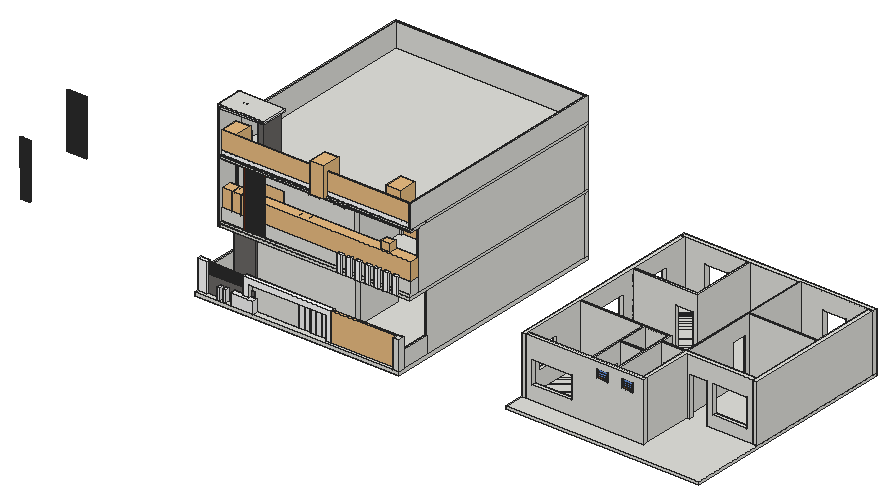
# SketchUp Ruby script. Lengths in inches.
U = 1.inch
M = Sketchup.active_model
def pt(a) = Geom::Point3d.new(a.map { |v| v * U })
def face(e, loops, mat)
  f = e.add_face(loops[0].map { |a| pt(a) })
  loops[1..].each { |l| e.add_face(l.map { |a| pt(a) }).erase! }
  f.material = f.back_material = mat if mat
  f
end
# faces: each face lists its corners as indices into pts; further lists are holes
def faces(e, pts, list, mat = nil) = list.each { |f| face(e, (f[0].is_a?(Array) ? f : [f]).map { |l| l.map { |i| pts[i] } }, mat) }
# xy, xz, yz: faces in a plane at the given z, y or x. An outline is a flat list of corners, or four numbers for a rectangle; further outlines are holes
def ring(l) = l.size == 4 ? [[l[0], l[1]], [l[2], l[1]], [l[2], l[3]], [l[0], l[3]]] : l.each_slice(2).to_a
def flat(e, list, mat, &to3) = list.each { |f| face(e, (f[0].is_a?(Array) ? f : [f]).map { |l| ring(l).map { |u, v| to3.(u, v) } }, mat) }
def xy(e, z, list, mat = nil) = flat(e, list, mat) { |x, y| [x, y, z] }
def xz(e, y, list, mat = nil) = flat(e, list, mat) { |x, z| [x, y, z] }
def yz(e, x, list, mat = nil) = flat(e, list, mat) { |y, z| [x, y, z] }
def lines(e, pts, list) = list.each { |a, b| e.add_line(pt(pts[a]), pt(pts[b])) }
# prism: a flat outline (further loops are holes) pulled along v
def prism(e, loops, v, mat = nil)
  f = face(e, loops, mat); d = Geom::Vector3d.new(v.map { |x| x * U })
  f.pushpull(f.normal.samedirection?(d) ? d.length : -d.length)
end
def box(e, o, s, mat = nil) = prism(e, [[o, [o[0] + s[0], o[1], o[2]], [o[0] + s[0], o[1] + s[1], o[2]], [o[0], o[1] + s[1], o[2]]]], [0, 0, s[2]], mat)
def at(x, y, z, deg = 0) = Geom::Transformation.translation(pt([x, y, z])) * Geom::Transformation.rotation(ORIGIN, Z_AXIS, deg.degrees)
def axes(o, x, y, z) = Geom::Transformation.new([*x, 0, *y, 0, *z, 0, *pt(o).to_a, 1])
def part(name) = M.definitions.add(name)
# library, detail: a bought-in or finely detailed component or shape, given as its bounding box
def library(name, o, s) = part(name).tap { |d| box(d.entities, o, s) }
def detail(e, o, s) = box(e.add_group.entities, o, s)
def put(e, d, t, mat = nil) = e.add_instance(d, t).tap { |i| i.material = mat if mat }
def group(e, t, mat = nil) = e.add_group.tap { |g| g.transformation = t; g.material = mat if mat }.entities
root = M.entities
M.materials.add("Paint Brown Gloss 1.5cm").color = [255, 255, 255]
M.materials.add("Polis06_194").color = [79, 50, 36]
M.materials.add("Stone C 250cm").color = [107, 104, 102]
M.materials.add("Tiles Marble White 03 180cm\#1").color = [241, 241, 241]
M.materials.add("Wood Dark 02 100cm").color = [99, 39, 19]
M.materials.add("Wood Mahogany 33-46 100cm").color = [84, 42, 21]
M.materials.add("[Translucent Glass Blue]").color = [100, 149, 237]
M.materials["[Translucent Glass Blue]"].alpha = 0.5
M.materials.add("[Translucent Glass Gray]").color = [128, 128, 128]
M.materials["[Translucent Glass Gray]"].alpha = 0.1
M.materials.add("[Wood Floor Parquet]").color = [145, 89, 39]
c1 = part("Stair step")
box(c1.entities,[0,0,0],[42,12,7])
c2 = part("ventilater")
prism(c2.entities,[[[2,7.78,8.95],[2,1.41,2.59],[2,0,4],[2,6.36,10.36]]],[20,0,0],"[Translucent Glass Blue]")
prism(c2.entities,[[[2,1.41,13.34],[22,1.41,13.34],[22,0,14.75],[2,0,14.75]]],[0,6.36,6.36],"[Translucent Glass Blue]")
prism(c2.entities,[[[2,1.41,7.96],[22,1.41,7.96],[22,0,9.375],[2,0,9.375]]],[0,6.36,6.36],"[Translucent Glass Blue]")
g1 = group(c2.entities,at(0,0,0))
xy(g1,0,[[0,0,24,9]],"[Wood Floor Parquet]")
xy(g1,2,[[2,0,22,9]],"[Wood Floor Parquet]")
xy(g1,22,[[2,0,22,9]],"[Wood Floor Parquet]")
xy(g1,24,[[0,0,24,9]],"[Wood Floor Parquet]")
xz(g1,0,[[[0,0,24,24],[2,2,22,22]]],"[Wood Floor Parquet]")
xz(g1,9,[[[0,0,24,24],[2,2,22,22]]],"[Wood Floor Parquet]")
yz(g1,0,[[0,0,9,24]],"[Wood Floor Parquet]")
yz(g1,2,[[0,2,9,22]],"[Wood Floor Parquet]")
yz(g1,22,[[0,2,9,22]])
yz(g1,24,[[0,0,9,24]],"[Wood Floor Parquet]")
c3 = library("PINTU 6 YA",[0,-0.6875,0],[35.83,8.07,80.71])
c4 = library("Flush door assembly",[0,0,0],[5.12,30.08,83.9375])
c5 = part("Flush door")
xy(c5.entities,0,[[0,0,4.72,1.18],[0,34.25,4.72,35.43]],"Polis06_194")
xy(c5.entities,85.26,[[0,1.18,4.72,34.25]],"Polis06_194")
xy(c5.entities,86.61,[[0,0,4.72,35.43]],"Polis06_194")
xz(c5.entities,0,[[0,0,4.72,86.61]],"Polis06_194")
xz(c5.entities,1.18,[[0,0,2.36,85.26],[2.36,0,4.72,85.26]],"Polis06_194")
xz(c5.entities,34.25,[[0,0,4.72,85.26]],"Polis06_194")
xz(c5.entities,35.43,[[0,0,4.72,86.61]],"Polis06_194")
yz(c5.entities,0,[[0,0,1.18,86.61],[34.25,0,35.43,86.61],[1.18,85.26,34.25,86.61]],"Polis06_194")
yz(c5.entities,2.36,[[1.18,0,34.25,0,34.25,85.21,1.18,85.26]],"Polis06_194")
yz(c5.entities,4.72,[[0,0,1.18,86.61],[34.25,0,35.43,86.61],[1.18,85.26,34.25,86.61]],"Polis06_194")
c6 = library("Untitled",[0,0,0],[36,4.39,84])
c7 = library("Window 46-12",[-37.28,-2.15,0],[74.56,4.3,92.91])
c8 = library("Window 46-47",[-61.02,-2.17,0],[122.04,4.34,74.02])
c9 = library("Window 46-15",[-34.06,-3.13,0],[68.12,6.24,59.06])
c10 = part("Flat panel")
box(c10.entities,[0,0,-1],[25,83.4375,1])
c11 = library("Round downlight",[0,0,-2.25],[6,6,4])
c12 = part("Square post")
box(c12.entities,[0,0,0],[1.8125,1.75,76.8125])
c13 = library("Garage Gate 243 111",[-105.76,-3.7,0],[211.52,7.4,101.23])
c14 = library("Potted Plant 02",[-16.98,-19.78,0],[30.04,38.68,37.52])
c15 = library("Potted Plant 13",[-10,-7.28,0],[18.93,15.17,39.22])
c16 = part("Group\#18")
p = [[1.37,4.61,43.28],[1.44,55.5625,43.28],[1.44,55.5625,4.4375],[1.37,4.61,4.4375]]
faces(c16.entities,p,[[0,1,2,3]],"[Translucent Glass Gray]")
g2 = group(c16.entities,at(0,0,0))
xy(g2,0,[[0.0625,0,2.5,60]])
xy(g2,3.125,[[0,3.125,0.59,56.875],[1.84,3.125,2.4375,56.875]])
xy(g2,4.4375,[[0.66,4.4375,1.91,55.5625]])
xy(g2,43.5625,[[0.66,4.4375,1.91,55.5625]])
xy(g2,44.875,[[0,3.125,0.59,56.875],[1.84,3.125,2.4375,56.875]])
xy(g2,48,[[0.0625,0,2.5,60]])
xz(g2,0,[[0.0625,0,2.5,48]])
xz(g2,3.125,[[0,3.125,0.59,44.875],[1.84,3.125,2.4375,44.875]])
xz(g2,4.4375,[[0.66,4.4375,1.91,43.5625]])
xz(g2,55.5625,[[0.66,4.4375,1.91,43.5625]])
xz(g2,56.875,[[0,3.125,0.59,44.875],[1.84,3.125,2.4375,44.875]])
xz(g2,60,[[0.0625,0,2.5,48]])
p = [[0,3.125,3.125],[0.0625,0,0],[0.0625,0,48],[0,3.125,44.875],[0,56.875,3.125],[0.0625,60,0],
  [2.5,0,0],[2.4375,3.125,3.125],[2.4375,3.125,44.875],[2.5,0,48],[2.5,60,0],[2.4375,56.875,3.125],
  [0,56.875,44.875],[0.0625,60,48],[2.5,60,48],[2.4375,56.875,44.875],[0.66,4.4375,4.4375],[0.59,3.125,3.125],
  [0.59,3.125,44.875],[0.66,4.4375,43.5625],[0.66,55.5625,4.4375],[0.59,56.875,3.125],[1.84,3.125,3.125],[1.91,4.4375,4.4375],
  [1.91,4.4375,43.5625],[1.84,3.125,44.875],[1.84,56.875,3.125],[1.91,55.5625,4.4375],[0.66,55.5625,43.5625],[0.59,56.875,44.875],
  [1.84,56.875,44.875],[1.91,55.5625,43.5625]]
faces(g2,p,[[0,1,2,3],[4,5,1,0],[6,7,8,9],[10,11,7,6],[12,13,5,4],[14,15,11,10],[16,17,18,19],[20,21,17,16],
  [22,23,24,25],[26,27,23,22],[28,29,21,20],[30,31,27,26],[19,18,29,28],[25,24,31,30],[3,2,13,12],[9,8,15,14]])
c17 = part("Group\#28")
xy(c17.entities,0,[[0,0,402.5,9]])
xy(c17.entities,36,[[51,0,99,9],[298.5,0,346.5,9]])
xy(c17.entities,84,[[51,0,99,9],[298.5,0,346.5,9]])
xy(c17.entities,120,[[0,0,402.5,9]])
xz(c17.entities,0,[[0,0,9,120],[[9,0,141,120],[51,36,99,84]],[141,0,145.5,120],[145.5,0,247,120],[247,0,251.5,120],
  [[251.5,0,393.5,120],[298.5,36,346.5,84]],[393.5,0,402.5,120]])
xz(c17.entities,9,[[[0,0,402.5,120],[51,36,99,84],[298.5,36,346.5,84]]])
yz(c17.entities,0,[[0,0,9,120]])
yz(c17.entities,51,[[0,36,9,84]])
yz(c17.entities,99,[[0,36,9,84]])
yz(c17.entities,298.5,[[0,36,9,84]])
yz(c17.entities,346.5,[[0,36,9,84]])
yz(c17.entities,402.5,[[0,0,9,120]])
c18 = part("Group\#29")
xy(c18.entities,0,[[0,0,9,416]])
xy(c18.entities,36,[[0,33,9,81],[0,183.5,9,255.5],[0,308,9,368]])
xy(c18.entities,84,[[0,33,9,81],[0,183.5,9,255.5],[0,308,9,368]])
xy(c18.entities,120,[[0,0,9,416]])
xz(c18.entities,0,[[0,0,9,120]])
xz(c18.entities,33,[[0,36,9,84]])
xz(c18.entities,81,[[0,36,9,84]])
xz(c18.entities,183.5,[[0,36,9,84]])
xz(c18.entities,255.5,[[0,36,9,84]])
xz(c18.entities,308,[[0,36,9,84]])
xz(c18.entities,368,[[0,36,9,84]])
xz(c18.entities,416,[[0,0,9,120]])
yz(c18.entities,0,[[[0,0,416,120],[183.5,36,255.5,84],[308,36,368,84],[33,36,81,84]]])
yz(c18.entities,9,[[0,0,9,120],[[9,0,141,120],[33,36,81,84]],[141,0,145.5,120],[[145.5,0,279.5,120],[183.5,36,255.5,84]],[279.5,0,284,120],
  [[284,0,416,120],[308,36,368,84]]])
c19 = part("Group\#30")
xy(c19.entities,0,[[0,0,246,9]])
xy(c19.entities,30,[[12,0,96,9]])
xy(c19.entities,78,[[12,0,96,9]])
xy(c19.entities,90,[[148.5,0,172.5,9],[201,0,225,9]])
xy(c19.entities,108,[[148.5,0,172.5,9],[201,0,225,9]])
xy(c19.entities,120,[[0,0,246,9]])
xz(c19.entities,0,[[[0,0,246,120],[12,30,96,78],[148.5,90,172.5,108],[201,90,225,108]]])
xz(c19.entities,9,[[[0,0,132,120],[12,30,96,78]],[132,0,136.5,120],[[136.5,0,184.5,120],[148.5,90,172.5,108]],[184.5,0,189,120],[[189,0,237,120],[201,90,225,108]],
  [237,0,246,120]])
yz(c19.entities,0,[[0,0,9,120]])
yz(c19.entities,12,[[0,30,9,78]])
yz(c19.entities,96,[[0,30,9,78]])
yz(c19.entities,148.5,[[0,90,9,108]])
yz(c19.entities,172.5,[[0,90,9,108]])
yz(c19.entities,201,[[0,90,9,108]])
yz(c19.entities,225,[[0,90,9,108]])
yz(c19.entities,246,[[0,0,9,120]])
c20 = part("Group\#33")
xy(c20.entities,0,[[0,0,90,4.5],[126,0,126,4.5,132,4.5,132,136.5,136.5,136.5,136.5,0]])
xy(c20.entities,84,[[90,0,126,4.5]])
xy(c20.entities,120,[[0,0,136.5,0,136.5,136.5,132,136.5,132,4.5,0,4.5]])
xz(c20.entities,0,[[0,0,90,0,90,84,126,84,126,0,136.5,0,136.5,120,0,120]])
xz(c20.entities,4.5,[[0,0,0,120,132,120,132,0,126,0,126,84,90,84,90,0]])
xz(c20.entities,136.5,[[132,0,136.5,120]])
yz(c20.entities,0,[[0,0,4.5,120]])
yz(c20.entities,90,[[0,0,4.5,84]])
yz(c20.entities,126,[[0,0,4.5,84]])
yz(c20.entities,132,[[4.5,0,136.5,120]])
yz(c20.entities,136.5,[[0,0,136.5,120]])
c21 = part("Group\#34")
xy(c21.entities,0,[[0,-157,4.55,-42],[0,-6,0,10.5,4.5,10.5,4.5,4.5,146.5,4.5,146.5,0,4.55,0,4.55,-6],[0,46.5,4.5,136.5]])
xy(c21.entities,84,[[0,-42,4.55,-6],[0,10.5,4.5,46.5]])
xy(c21.entities,120,[[0,-157,4.55,-157,4.55,0,146.5,0,146.5,4.5,4.5,4.5,4.5,136.5,0,136.5]])
xz(c21.entities,-157,[[0,0,4.55,120]])
xz(c21.entities,-42,[[0,0,4.55,84]])
xz(c21.entities,-6,[[0,0,4.55,84]])
xz(c21.entities,0,[[4.55,0,146.5,120]])
xz(c21.entities,4.5,[[4.5,0,146.5,120]])
xz(c21.entities,10.5,[[0,0,4.5,84]])
xz(c21.entities,46.5,[[0,0,4.5,84]])
xz(c21.entities,136.5,[[0,0,4.5,120]])
yz(c21.entities,0,[[-157,0,-157,120,136.5,120,136.5,0,46.5,0,46.5,84,10.5,84,10.5,0,-6,0,-6,84,-42,84,-42,0]])
yz(c21.entities,4.5,[[4.5,0,10.5,0,10.5,84,46.5,84,46.5,0,136.5,0,136.5,120,4.5,120]])
yz(c21.entities,4.55,[[-157,0,-42,0,-42,84,-6,84,-6,0,0,0,0,120,-157,120]])
yz(c21.entities,146.5,[[0,0,4.5,120]])
c22 = part("Group\#38")
xy(c22.entities,0,[[184.5,0,184.5,66,136.5,66,136.5,60,132,60,132,132,126,132,126,136.5,154.5,136.5,154.5,132,136.5,132,136.5,70.5,184.5,70.5,184.5,132,178.5,132,178.5,136.5,189,136.5,189,0],[132,0,136.5,30],[0,132,90,136.5]])
xy(c22.entities,84,[[132,30,136.5,60],[90,132,126,136.5],[154.5,132,178.5,136.5]])
xy(c22.entities,120,[[[132,0,136.5,0,136.5,66,184.5,66,184.5,0,189,0,189,136.5,0,136.5,0,132,132,132],[136.5,70.5,184.5,132]]])
xz(c22.entities,0,[[132,0,136.5,120],[184.5,0,189,120]])
xz(c22.entities,30,[[132,0,136.5,84]])
xz(c22.entities,60,[[132,0,136.5,84]])
xz(c22.entities,66,[[136.5,0,184.5,120]])
xz(c22.entities,70.5,[[136.5,0,184.5,120]])
xz(c22.entities,132,[[0,0,90,0,90,84,126,84,126,0,132,0,132,120,0,120],[136.5,0,154.5,0,154.5,84,178.5,84,178.5,0,184.5,0,184.5,120,136.5,120]])
xz(c22.entities,136.5,[[0,0,0,120,189,120,189,0,178.5,0,178.5,84,154.5,84,154.5,0,126,0,126,84,90,84,90,0]])
yz(c22.entities,0,[[132,0,136.5,120]])
yz(c22.entities,90,[[132,0,136.5,84]])
yz(c22.entities,126,[[132,0,136.5,84]])
yz(c22.entities,132,[[0,0,0,120,132,120,132,0,60,0,60,84,30,84,30,0]])
yz(c22.entities,136.5,[[0,0,30,0,30,84,60,84,60,0,66,0,66,120,0,120],[70.5,0,132,120]])
yz(c22.entities,154.5,[[132,0,136.5,84]])
yz(c22.entities,178.5,[[132,0,136.5,84]])
yz(c22.entities,184.5,[[0,0,66,120],[70.5,0,132,120]])
yz(c22.entities,189,[[0,0,136.5,120]])
c23 = part("Group\#39")
prism(c23.entities,[[[6,4.5,0],[0,4.5,0],[0,4.5,120],[48,4.5,120],[48,4.5,0],[30,4.5,0],[30,4.5,84],[6,4.5,84]]],[0,-4.5,0])
c24 = part("Group\#31")
xy(c24.entities,0,[[0,0,0,113.5,15,113.5,15,104.5,9,104.5,9,0],[51,104.5,147.5,113.5]])
xy(c24.entities,24,[[63.5,104.5,135.5,113.5]])
xy(c24.entities,84,[[15,104.5,51,113.5],[63.5,104.5,135.5,113.5]])
xy(c24.entities,120,[[0,0,9,0,9,104.5,147.5,104.5,147.5,113.5,0,113.5]])
xz(c24.entities,0,[[0,0,9,120]])
xz(c24.entities,104.5,[[[9,0,15,0,15,84,51,84,51,0,147.5,0,147.5,120,9,120],[63.5,24,135.5,84]]])
xz(c24.entities,113.5,[[[0,0,0,120,147.5,120,147.5,0,51,0,51,84,15,84,15,0],[63.5,24,135.5,84]]])
yz(c24.entities,0,[[0,0,113.5,120]])
yz(c24.entities,9,[[0,0,104.5,120]])
yz(c24.entities,15,[[104.5,0,113.5,84]])
yz(c24.entities,51,[[104.5,0,113.5,84]])
yz(c24.entities,63.5,[[104.5,24,113.5,84]])
yz(c24.entities,135.5,[[104.5,24,113.5,84]])
yz(c24.entities,147.5,[[104.5,0,113.5,120]])
c25 = part("Group\#19")
p = [[0.77,2.6,2.4375],[0.77,2.6,45.4375],[0.76,69.5625,45.4375],[0.76,69.5625,2.4375]]
faces(c25.entities,p,[[0,1,2,3]],"[Translucent Glass Gray]")
g3 = group(c25.entities,at(0,0,0))
xy(g3,0,[[0,0,1.5,72]])
xy(g3,1.6875,[[0,1.6875,0.32,70.3125],[1.13,1.6875,1.5,70.3125]])
xy(g3,2.4375,[[0.32,2.4375,1.13,69.5625]])
xy(g3,45.5625,[[0.32,2.4375,1.13,69.5625]])
xy(g3,46.3125,[[0,1.6875,0.32,70.3125],[1.13,1.6875,1.5,70.3125]])
xy(g3,48,[[0,0,1.5,72]])
xz(g3,0,[[0,0,1.5,48]])
xz(g3,1.6875,[[0,1.6875,0.32,46.3125],[1.13,1.6875,1.5,46.3125]])
xz(g3,2.4375,[[0.32,2.4375,1.13,45.5625]])
xz(g3,69.5625,[[0.32,2.4375,1.13,45.5625]])
xz(g3,70.3125,[[0,1.6875,0.32,46.3125],[1.13,1.6875,1.5,46.3125]])
xz(g3,72,[[0,0,1.5,48]])
yz(g3,0,[[[0,0,72,48],[1.6875,1.6875,70.3125,46.3125]]])
yz(g3,0.32,[[[1.6875,1.6875,70.3125,46.3125],[2.4375,2.4375,69.5625,45.5625]]])
yz(g3,1.13,[[[1.6875,1.6875,70.3125,46.3125],[2.4375,2.4375,69.5625,45.5625]]])
yz(g3,1.5,[[[0,0,72,48],[1.6875,1.6875,70.3125,46.3125]]])
c26 = part("Group\#40")
p = [[44.3125,1.21,43.61],[44.3125,1.21,3.6875],[3.84,1.24,3.6875],[3.84,1.24,43.61]]
faces(c26.entities,p,[[0,1,2,3]],"[Translucent Glass Gray]")
g4 = group(c26.entities,at(0,0,0))
xy(g4,0,[[0,0,48,2.6875]])
xy(g4,2.4375,[[2.4375,0,45.5625,0.78],[2.4375,1.85,45.5625,2.6875]])
xy(g4,3.6875,[[3.6875,0.78,44.3125,1.85]])
xy(g4,44.3125,[[3.6875,0.78,44.3125,1.85]])
xy(g4,45.5625,[[2.4375,0,45.5625,0.78],[2.4375,1.85,45.5625,2.6875]])
xy(g4,48,[[0,0,48,2.6875]])
xz(g4,0,[[[0,0,48,48],[2.4375,2.4375,45.5625,45.5625]]])
xz(g4,0.78,[[[2.4375,2.4375,45.5625,45.5625],[3.6875,3.6875,44.3125,44.3125]]])
xz(g4,1.85,[[[2.4375,2.4375,45.5625,45.5625],[3.6875,3.6875,44.3125,44.3125]]])
xz(g4,2.6875,[[[0,0,48,48],[2.4375,2.4375,45.5625,45.5625]]])
yz(g4,0,[[0,0,2.6875,48]])
yz(g4,2.4375,[[0,2.4375,0.78,45.5625],[1.85,2.4375,2.6875,45.5625]])
yz(g4,3.6875,[[0.78,3.6875,1.85,44.3125]])
yz(g4,44.3125,[[0.78,3.6875,1.85,44.3125]])
yz(g4,45.5625,[[0,2.4375,0.78,45.5625],[1.85,2.4375,2.6875,45.5625]])
yz(g4,48,[[0,0,2.6875,48]])
c27 = part("Round rod")
prism(c27.entities,[[[1.11,0.71,0],[1.125,0.5625,0],[1.11,0.42,0],[1.05,0.28,0],[0.96,0.16,0],[0.84,0.08,0],[0.71,0.02,0],[0.5625,0,0],[0.42,0.02,0],[0.28,0.08,0],[0.16,0.16,0],[0.08,0.28,0],[0.02,0.42,0],[0,0.5625,0],[0.02,0.71,0],[0.08,0.84,0],[0.16,0.96,0],[0.28,1.05,0],[0.42,1.11,0],[0.5625,1.125,0],[0.71,1.11,0],[0.84,1.05,0],[0.96,0.96,0],[1.05,0.84,0]]],[0,0,24])
c28 = library("Group\#45",[0,0,0],[399.29,21.95,36.98])
c29 = part("Vertical batten")
prism(c29.entities,[[[0,0.125,0],[1.6875,0.125,0],[1.6875,-0.5,0],[0,-0.5,0]]],[0,-0.125,115])
c30 = part("Group\#59")
xy(c30.entities,0,[[0,0.125,21.3,0.4375]])
xy(c30.entities,115,[[0,0,21.3,0.3125]])
yz(c30.entities,0,[[0.125,0,0,115,0.3125,115,0.4375,0]])
yz(c30.entities,21.3,[[0.125,0,0.4375,0,0.3125,115,0,115]])
p = [[21.3,0,115],[0.625,0,115],[0.625,0.125,0],[21.3,0.125,0],[0,0.3125,115],[21.3,0.3125,115],
  [21.3,0.4375,0],[0,0.4375,0]]
faces(c30.entities,p,[[0,1,2,3],[4,5,6,7]])
put(c30.entities,c29,at(0,0,0))
put(c30.entities,c29,at(3.92,0,0))
put(c30.entities,c29,at(7.85,0,0))
put(c30.entities,c29,at(11.77,0,0))
put(c30.entities,c29,at(15.69,0,0))
put(c30.entities,c29,at(19.61,0,0))
c31 = part("Group\#61")
prism(c31.entities,[[[9.625,2.75,0],[9.625,2.75,33.375],[9.625,7.8125,33.375],[9.625,8.875,33.375],[9.625,8.875,36.5625],[9.625,0,36.5625],[9.625,0,0]]],[-9.625,0,0])
c32 = library("Group\#62",[0,0,0],[397.4375,3.15,36.98])
box(root,[335.52,145.54,347.82],[95.87,55.93,0.79])
box(root,[413.77,151.7,252],[12,45.8,89.625],"Stone C 250cm")
prism(root,[[[311.52,611.04,0],[335.52,611.04,0],[335.52,606.54,0],[316.02,606.54,0],[316.02,132.1,0],[311.52,132.1,0]]],[0,0,36])
xy(root,-6.5625,[[947.33,195.04,1079.33,327.04],[1083.83,195.04,1131.83,261.04],[1083.83,265.54,1131.83,327.04],[947.33,470.04,1079.33,602.04],[1189.83,470.04,1331.83,602.04]])
xy(root,0,[[726.02,116.04,738.02,128.04],[733.52,128.04,738.02,188.04],[733.52,188.04,738.02,378.54],[344.52,197.04,476.52,329.04],[481.02,197.04,529.02,263.04],
  [481.02,267.54,476.52,329.04,529.02,329.04,529.02,267.54],[587.02,387.54,729.02,465.54],[344.52,470.04,476.52,602.04],[587.02,470.04,729.02,602.04]])
xy(root,36,[[733.52,128.04,738.02,188.04]])
xy(root,60,[[726.02,116.04,738.02,128.04]])
xy(root,126,[[344.52,195.04,476.52,327.04],[481.02,195.04,529.02,261.04],[481.02,265.54,529.02,327.04],[344.52,470.04,476.52,602.04],[587.02,470.04,729.02,602.04]])
xy(root,131,[[481.02,267.54,529.02,267.54,529.02,329.04,476.52,329.04]])
xy(root,252,[[340.02,145.54,738.02,146.54],[340.02,146.54,733.52,150.04],[733.52,146.54,738.02,611.04],[335.52,606.54,733.52,611.04]])
xy(root,255,[[340.02,145.54,738.02,146.54]])
xy(root,264,[[340.02,146.54,733.52,148.29],[340.02,148.29,733.52,150.04]])
xy(root,300.98,[[733.52,146.54,738.02,611.04],[335.52,606.54,733.52,611.04]])
xz(root,116.04,[[726.02,0,738.02,60]])
xz(root,128.04,[[726.02,0,733.52,60],[733.52,0,738.02,36],[733.52,36,738.02,60]])
xz(root,145.54,[[340.02,252,738.02,255]])
xz(root,146.54,[[340.02,252,733.52,255],[733.52,252,738.02,255],[733.52,255,738.02,300.98]])
xz(root,146.54,[[340.02,255,733.52,264]],"Paint Brown Gloss 1.5cm")
xz(root,150.04,[[340.02,252,733.52,264]])
xz(root,188.04,[[733.52,0,738.02,36]])
xz(root,267.54,[[481.02,0,529.02,131]])
xz(root,329.04,[[476.52,0,529.02,131]])
xz(root,606.54,[[335.52,252,733.52,300.98]])
xz(root,611.04,[[335.52,252,733.52,300.98],[733.52,252,738.02,300.98]])
yz(root,335.52,[[606.54,252,201.47,252.15,201.49,301.14,606.55,300.99,606.55,300.98,606.54,300.98],[606.54,252,606.54,300.98,606.55,300.98],[606.54,252,606.55,300.98,611.04,300.98,611.04,252]])
yz(root,340.02,[[145.54,252,146.54,255],[146.54,252,150.04,264],[606.54,252,606.55,300.99,201.49,301.14,201.47,252.15]])
yz(root,529.02,[[267.54,0,329.04,131]])
yz(root,726.02,[[116.04,0,128.04,60]])
yz(root,733.52,[[128.04,0,188.04,36],[146.54,252,150.04,264],[150.04,252,606.54,300.98],[606.54,252,611.04,300.98],[146.54,264,150.04,300.98]])
yz(root,738.02,[[116.04,0,128.04,60],[128.04,0,188.04,36],[145.54,252,146.54,255],[146.54,252,611.04,300.98]])
p = [[476.52,329.04,0],[481.02,267.54,0],[481.02,267.54,126],[481.02,267.54,131],[476.52,329.04,131],[335.52,201.47,252.15],
  [335.52,606.54,252],[340.02,606.54,252],[340.02,201.47,252.15],[335.52,606.55,300.98],[335.52,606.55,300.99],[340.02,606.55,300.99],
  [340.02,201.49,301.14],[335.52,201.49,301.14],[523.02,537.27,0],[523.02,537.54,0],[582.52,537.27,0],[582.52,537.54,0],
  [340.02,305.04,36],[340.02,233.04,36],[340.02,233.04,84],[340.02,305.04,84],[340.02,369.54,84],[340.02,441.54,84],
  [340.02,441.54,36],[340.02,369.54,36],[340.02,494.04,84],[340.02,554.04,84],[340.02,554.04,36],[340.02,494.04,36],
  [434.52,606.54,36],[434.52,606.54,84],[386.52,606.54,84],[386.52,606.54,36],[735.52,150.6,155],[735.77,168.99,155],
  [656.42,150.6,155],[435.56,147.66,131],[435.56,145.54,131],[388.23,145.54,131],[388.23,147.66,131]]
faces(root,p,[[0,1,2,3,4],[5,6,7,8],[7,6,9,10,11],[5,8,12,13],[10,13,12,11]])
lines(root,p,[[14,15],[16,17],[18,19],[19,20],[20,21],[21,18],[22,23],[23,24],[24,25],[25,22],[26,27],[27,28],
  [28,29],[29,26],[30,31],[31,32],[32,33],[33,30],[34,35],[36,34],[37,38],[39,40],[40,37]])
put(root,c1,at(481.02,471.25,0))
put(root,c1,at(481.02,483.25,7))
put(root,c1,at(481.02,495.25,14))
put(root,c1,at(481.02,507.25,21))
put(root,c1,at(481.02,519.25,28))
put(root,c1,at(481.02,531.25,35))
put(root,c1,at(481.02,543.25,42))
put(root,c1,at(481.02,555.25,49))
put(root,c1,at(481.02,567.25,56))
put(root,c1,axes([481.02,579.25,63],[2.41667,0,0],[0,1.89926,0],[0,0,1]))
put(root,c2,axes([493.2,189.66,90],[0.99237,0,0],[0,0.67,0],[0,0,0.75]))
put(root,c2,axes([547.95,189.66,90],[0.99237,0,0],[0,0.67,0],[0,0,0.75]))
put(root,c3,axes([434.52,467.79,0],[1.00475,0,0],[0,1,0],[0,0,1.04078]))
put(root,c3,axes([470.52,331.29,0],[-1.00475,0,0],[0,-1,0],[0,0,1.04078]))
put(root,c3,axes([588.71,476.04,0],[0,1.00475,0],[-1,0,0],[0,0,1.04078]))
put(root,c4,at(583.59,435.54,0))
put(root,c5,axes([477.17,227.04,0],[0.69,0,0],[0,0.83111,0],[0,0,0.96982]))
put(root,c5,axes([499.02,329.04,0],[0,-0.3594,0],[0.84667,0,0],[0,0,0.96982]))
put(root,c5,axes([539.52,297.54,-2.57],[0,-1.47625,0],[0.84667,0,0],[0,0,1]))
put(root,c1,at(540.57,567.25,70))
put(root,c2,axes([1096.02,187.66,83.4375],[0.99237,0,0],[0,0.67,0],[0,0,0.75]))
put(root,c2,axes([1148.33,187.66,83.4375],[0.99237,0,0],[0,0.67,0],[0,0,0.75]))
put(root,c2,axes([493.2,187.66,216],[0.99237,0,0],[0,0.67,0],[0,0,0.75]))
put(root,c2,axes([545.52,187.66,216],[0.99237,0,0],[0,0.67,0],[0,0,0.75]))
put(root,c1,at(540.57,555.25,77))
put(root,c1,at(540.57,543.25,84))
put(root,c1,at(540.57,531.25,91))
put(root,c1,at(540.57,519.25,98))
put(root,c1,at(537.3,515.54,119))
put(root,c3,axes([588.71,476.04,124.625],[0,1.00475,0],[-1,0,0],[0,0,1.04078]))
put(root,c3,axes([588.71,423.54,124.625],[0,1.00475,0],[-1,0,0],[0,0,1.04078]))
put(root,c3,axes([434.52,467.79,124.625],[1.00475,0,0],[0,1,0],[0,0,1.04078]))
put(root,c3,axes([434.52,325.35,126],[1.00475,0,0],[0,1,0],[0,0,1.04078]))
put(root,c5,axes([539.52,306.29,126],[0,-0.77415,0],[0.67733,0,0],[0,0,0.96982]))
put(root,c5,axes([499.02,329.29,126],[0,-0.77415,0],[0.67733,0,0],[0,0,0.96982]))
put(root,c5,axes([478.77,225.04,126],[0.77415,0,0],[0,0.84667,0],[0,0,0.96982]))
put(root,c6,at(596.52,304.04,126))
put(root,c7,axes([681.02,300.8,150],[0.96557,0,0],[0,-0.58709,0],[0,0,0.64576]))
put(root,c8,axes([398.52,190.54,155.875],[0.68826,0,0],[0,0.4,0],[0,0,0.65021]))
put(root,c9,axes([658.02,382.625,36],[0.70474,0,0],[0,0.6847,0],[0,0,0.82]))
put(root,c10,at(628.05,223.31,246,-90),"Wood Mahogany 33-46 100cm")
put(root,c10,at(628.05,262.99,246,-90),"Wood Mahogany 33-46 100cm")
put(root,c11,at(638.36,213.81,245,-90))
put(root,c11,at(638.36,253.49,245,-90))
put(root,c11,at(694.23,253.49,245,-90))
put(root,c11,at(694.23,213.81,245,-90))
put(root,c12,axes([329.52,126.75,56.99],[0,1,0],[0,0,1],[1,0,0]))
put(root,c12,axes([329.52,126.75,52.7],[0,1,0],[0,0,1],[1,0,0]))
put(root,c12,axes([329.52,126.75,48.42],[0,1,0],[0,0,1],[1,0,0]))
put(root,c12,axes([329.52,126.75,44.14],[0,1,0],[0,0,1],[1,0,0]))
put(root,c12,axes([329.52,126.75,39.86],[0,1,0],[0,0,1],[1,0,0]))
put(root,c13,axes([658.27,125.67,0],[0.6406,0,0],[0,0.64,0],[0,0,0.59269]))
put(root,c14,axes([357.875,168.03,252],[1,0,0],[0,1,0],[0,0,1.29099]))
put(root,c14,at(357.03,171.1875,253.28))
put(root,c14,axes([549.15,159.54,252],[1,0,0],[0,1,0],[0,0,1.63434]))
put(root,c14,axes([699.32,171.82,255.125],[1,0,0],[0,1,0],[0,0,1.6]))
put(root,c15,at(372.52,156.5,152.73))
put(root,c15,at(506.77,160.82,151.41))
put(root,c15,axes([680.45,160.82,148.85],[1,0,0],[0,1,0],[0,0,1.47]))
g5 = group(root,at(335.52,188.04,-6.5625))
box(g5,[-24,-72,0],[426.5,495,6.5625])
g6 = group(root,at(335.52,602.04,0))
xy(g6,-0.125,[[0,0,402.5,9]])
xy(g6,36,[[51,0,99,9]])
xy(g6,84,[[51,0,99,9]])
xy(g6,120,[[0,0,402.5,9]])
xz(g6,0,[[0,-0.125,9,120],[[9,-0.125,141,120],[51,36,99,84]],[141,-0.125,145.5,120],[145.5,-0.125,247,120],[247,-0.125,251.5,120],
  [251.5,-0.125,393.5,120],[393.5,-0.125,402.5,120]])
xz(g6,9,[[[0,-0.125,402.5,120],[51,36,99,84]]])
yz(g6,0,[[0,-0.125,9,120]])
yz(g6,51,[[0,36,9,84]])
yz(g6,99,[[0,36,9,84]])
yz(g6,402.5,[[0,-0.125,9,120]])
g7 = group(root,at(581.52,197.04,0))
box(g7,[0,0,0],[9,100.5,120])
g8 = group(root,at(529.02,197.04,0))
prism(g8,[[[0,66,0],[0,70.5,0],[0,132,0],[0,136.5,0],[4.5,136.5,0],[4.5,0,0],[0,0,0]]],[0,0,120])
g9 = group(root,at(476.52,197.04,0))
xy(g9,0,[[0,0,4.5,30],[0,60,4.5,132]])
xy(g9,84,[[0,30,4.5,60]])
xy(g9,120,[[0,0,4.5,132]])
xz(g9,0,[[0,0,4.5,120]])
xz(g9,30,[[0,0,4.5,84]])
xz(g9,60,[[0,0,4.5,84]])
xz(g9,132,[[0,0,4.5,120]])
yz(g9,0,[[0,0,0,120,132,120,132,0,60,0,60,84,30,84,30,0]])
yz(g9,4.5,[[0,0,30,0,30,84,60,84,60,0,66,0,66,120,0,120],[66,0,70.5,120],[70.5,0,132,120]])
g10 = group(root,at(481.02,263.04,0))
box(g10,[0,0,0],[48,4.5,120])
g11 = group(root,at(476.52,470.04,0))
box(g11,[0,0,0],[4.5,132,120])
g12 = group(root,at(344.52,465.54,0))
xy(g12,0,[[0,0,90,4.5],[126,0,136.5,4.5]])
xy(g12,84,[[90,0,126,4.5]])
xy(g12,120,[[0,0,136.5,4.5]])
xz(g12,0,[[0,0,90,0,90,84,126,84,126,0,136.5,0,136.5,120,0,120]])
xz(g12,4.5,[[0,0,0,120,132,120,132,0,126,0,126,84,90,84,90,0],[132,0,136.5,120]])
yz(g12,0,[[0,0,4.5,120]])
yz(g12,90,[[0,0,4.5,84]])
yz(g12,126,[[0,0,4.5,84]])
yz(g12,136.5,[[0,0,4.5,120]])
g13 = group(root,at(582.52,378.54,0))
xy(g13,0,[[151,-190.5,151,0,0,0,0,57,4.5,57,4.5,9,146.5,9,146.5,87,0,87,0,97.5,4.5,97.5,4.5,91.5,146.5,91.5,146.5,223.5,155.5,223.5,155.5,-190.5],[0,133.5,4.5,223.5]])
xy(g13,36,[[51.5,0,99.5,9]])
xy(g13,84,[[51.5,0,99.5,9],[0,57,4.5,87],[0,97.5,4.5,133.5]])
xy(g13,120,[[[151,-190.5,155.5,-190.5,155.5,223.5,146.5,223.5,146.5,91.5,4.5,91.5,4.5,223.5,0,223.5,0,0,151,0],[4.5,9,146.5,87]]])
xz(g13,-190.5,[[151,0,155.5,120]])
xz(g13,0,[[[0,0,151,120],[51.5,36,99.5,84]]])
xz(g13,9,[[[4.5,0,146.5,120],[51.5,36,99.5,84]]])
xz(g13,57,[[0,0,4.5,84]])
xz(g13,87,[[0,0,146.5,0,146.5,120,4.5,120,4.5,84,0,84]])
xz(g13,91.5,[[4.5,0,146.5,120]])
xz(g13,97.5,[[0,0,4.5,84]])
xz(g13,133.5,[[0,0,4.5,84]])
xz(g13,223.5,[[0,0,4.5,120],[146.5,0,155.5,120]])
yz(g13,0,[[0,0,0,120,223.5,120,223.5,0,133.5,0,133.5,84,97.5,84,97.5,0,87,0,87,84,57,84,57,0]])
yz(g13,4.5,[[9,0,57,0,57,84,87,84,87,120,9,120],[91.5,0,97.5,0,97.5,84,133.5,84,133.5,0,223.5,0,223.5,120,91.5,120]])
yz(g13,51.5,[[0,36,9,84]])
yz(g13,99.5,[[0,36,9,84]])
yz(g13,146.5,[[9,0,87,120],[91.5,0,223.5,120]])
yz(g13,151,[[-190.5,0,0,120]])
yz(g13,155.5,[[-190.5,0,223.5,120]])
g14 = group(root,at(344.52,188.04,0))
xy(g14,0,[[0,0,246,9]])
xy(g14,90,[[148.5,0,172.5,9],[203.25,0,227.25,9]])
xy(g14,108,[[148.5,0,172.5,9],[203.25,0,227.25,9]])
xy(g14,120,[[0,0,246,9]])
xz(g14,0,[[[0,0,246,120],[148.5,90,172.5,108],[203.25,90,227.25,108]]])
xz(g14,9,[[0,0,132,120],[132,0,136.5,120],[[136.5,0,184.5,120],[148.5,90,172.5,108]],[[184.5,0,246,120],[203.25,90,227.25,108]]])
yz(g14,0,[[0,0,9,120]])
yz(g14,148.5,[[0,90,9,108]])
yz(g14,172.5,[[0,90,9,108]])
yz(g14,203.25,[[0,90,9,108]])
yz(g14,227.25,[[0,90,9,108]])
yz(g14,246,[[0,0,9,120]])
g15 = group(root,at(533.52,293.04,0))
prism(g15,[[[48,4.5,0],[36,4.5,0],[36,4.5,84],[6,4.5,84],[6,4.5,0],[0,4.5,0],[0,4.5,120],[48,4.5,120]]],[0,-4.5,0])
g16 = group(root,at(344.52,329.04,0))
xy(g16,0,[[0,0,90,4.5],[126,0,154.5,4.5]])
xy(g16,84,[[90,0,126,4.5],[154.5,0,184.5,4.5]])
xy(g16,120,[[0,0,184.5,4.5]])
xz(g16,0,[[0,0,90,0,90,84,126,84,126,0,132,0,132,120,0,120],[132,0,154.5,0,154.5,84,184.5,84,184.5,120,132,120]])
xz(g16,4.5,[[0,0,0,120,184.5,120,184.5,84,154.5,84,154.5,0,126,0,126,84,90,84,90,0]])
yz(g16,0,[[0,0,4.5,120]])
yz(g16,90,[[0,0,4.5,84]])
yz(g16,126,[[0,0,4.5,84]])
yz(g16,154.5,[[0,0,4.5,84]])
yz(g16,184.5,[[0,84,4.5,120]])
g17 = group(root,at(338.82,233.04,36))
p = [[1.4,5.97,5.97],[1.4,5.97,41.96],[1.32,66.03,41.96],[1.32,66.03,5.97]]
faces(g17,p,[[0,1,2,3]],"[Translucent Glass Gray]")
g18 = group(g17,at(0,0,0))
xy(g18,0,[[0,0,2.5625,72]])
xy(g18,4.15,[[0,4.15,0.72,67.85],[1.84,4.15,2.5625,67.85]])
xy(g18,5.97,[[0.72,5.97,1.84,66.03]])
xy(g18,42.03,[[0.72,5.97,1.84,66.03]])
xy(g18,43.85,[[0,4.15,0.72,67.85],[1.84,4.15,2.5625,67.85]])
xy(g18,48,[[0,0,2.5625,72]])
xz(g18,0,[[0,0,2.5625,48]])
xz(g18,4.15,[[0,4.15,0.72,43.85],[1.84,4.15,2.5625,43.85]])
xz(g18,5.97,[[0.72,5.97,1.84,42.03]])
xz(g18,66.03,[[0.72,5.97,1.84,42.03]])
xz(g18,67.85,[[0,4.15,0.72,43.85],[1.84,4.15,2.5625,43.85]])
xz(g18,72,[[0,0,2.5625,48]])
yz(g18,0,[[[0,0,72,48],[4.15,4.15,67.85,43.85]]])
yz(g18,0.72,[[[4.15,4.15,67.85,43.85],[5.97,5.97,66.03,42.03]]])
yz(g18,1.84,[[[4.15,4.15,67.85,43.85],[5.97,5.97,66.03,42.03]]])
yz(g18,2.5625,[[[0,0,72,48],[4.15,4.15,67.85,43.85]]])
g19 = group(root,at(335.52,188.04,0))
xy(g19,0,[[0,0,9,414]])
xy(g19,36,[[0,45,9,117],[0,181.5,9,253.5],[0,306,9,366]])
xy(g19,84,[[0,45,9,117],[0,181.5,9,253.5],[0,306,9,366]])
xy(g19,120,[[0,0,9,414]])
xz(g19,0,[[0,0,9,120]])
xz(g19,45,[[0,36,9,84]])
xz(g19,117,[[0,36,9,84]])
xz(g19,181.5,[[0,36,9,84]])
xz(g19,253.5,[[0,36,9,84]])
xz(g19,306,[[0,36,9,84]])
xz(g19,366,[[0,36,9,84]])
xz(g19,414,[[0,0,9,120]])
yz(g19,0,[[[0,0,414,120],[45,36,117,84],[181.5,36,253.5,84],[306,36,366,84]]])
yz(g19,9,[[0,0,9,120],[[9,0,141,120],[45,36,117,84]],[141,0,145.5,120],[[145.5,0,277.5,120],[181.5,36,253.5,84]],[277.5,0,282,120],
  [[282,0,414,120],[306,36,366,84]]])
put(root,c16,at(339.51,494.04,36))
g20 = group(root,at(938.33,145.54,-12.5625))
box(g20,[0,0,0],[402.5,465.5,6])
put(root,c17,at(938.33,602.04,-6.5625))
put(root,c18,at(938.33,186.04,-6.5625))
put(root,c19,at(947.33,186.04,-6.5625))
g21 = group(root,at(1331.83,299.54,-6.5625))
prism(g21,[[[9,302.5,0],[9,0,0],[0,0,0],[0,9,0],[0,166,0],[0,170.5,0],[0,302.5,0]]],[0,0,120])
put(root,c20,at(947.33,465.54,-6.5625))
put(root,c21,at(1185.33,465.54,-6.5625))
put(root,c22,at(947.33,195.04,-6.5625))
put(root,c23,at(1136.33,304.04,-6.5625))
put(root,c24,at(1184.33,195.04,-6.5625))
put(root,c18,at(335.52,186.04,126))
put(root,c21,at(582.52,465.54,126))
put(root,c20,at(344.52,465.54,126))
put(root,c23,at(533.52,304.04,126))
g22 = group(root,at(335.52,145.54,120))
xy(g22,0,[[[0,0,402.5,465.5],[145.5,342.6875,147.625,342.6875,147.625,370,244,370,244,342.6875,247,342.6875,247,456.5,145.5,456.5]],[145.5,342.6875,145.5,456.5,247,456.5,247,342.6875,244,342.6875,244,454.5,147.625,454.5,147.625,342.6875]])
xy(g22,6,[[[0,0,402.5,0,402.5,23.46,398,23.46,398,154,402.5,154,402.5,465.5,0,465.5],[147.625,370,244,454.5]],[398,23.46,402.5,154]])
xz(g22,0,[[0,0,402.5,6]])
xz(g22,370,[[147.625,0,244,6]])
xz(g22,454.5,[[147.625,0,244,6]])
xz(g22,465.5,[[0,0,402.5,6]])
yz(g22,0,[[0,0,465.5,6]])
yz(g22,147.625,[[370,0,454.5,6]])
yz(g22,244,[[370,0,454.5,6]])
yz(g22,402.5,[[0,0,465.5,6]])
put(root,c17,at(335.52,602.04,126))
put(root,c19,at(344.52,186.04,126))
put(root,c22,at(344.52,195.04,126))
g23 = group(root,at(729.02,299.54,126))
prism(g23,[[[9,302.5,0],[9,-130.54,0],[4.5,-130.54,0],[4.5,0,0],[0,0,0],[0,9,0],[0,166,0],[0,170.5,0],[0,302.5,0]]],[0,0,120])
put(root,c24,at(581.52,195.04,126))
put(root,c25,at(338.62,369.54,36))
put(root,c25,at(340.93,369.54,162))
put(root,c16,at(339.96,494.04,162))
put(root,c26,at(386.52,605.96,36))
put(root,c26,at(386.52,603.85,162))
put(root,c26,at(634.02,603.85,162))
g24 = group(root,at(335.52,145.54,246))
xy(g24,0,[[4.5,2,4.5,40.875,0,40.875,0,465.5,402.5,465.5,402.5,2]])
xy(g24,3,[[4.5,0,402.5,2]])
xy(g24,6,[[4.5,0,402.5,0,402.5,465.5,0,465.5,0,40.875,4.5,40.875]])
xz(g24,0,[[4.5,3,402.5,6]])
xz(g24,2,[[4.5,0,402.5,3]])
xz(g24,40.875,[[0,0,4.5,6]])
xz(g24,465.5,[[0,0,402.5,6]])
yz(g24,0,[[40.875,0,465.5,6]])
yz(g24,4.5,[[2,0,2,3,0,3,0,6,40.875,6,40.875,0]])
yz(g24,402.5,[[2,0,465.5,0,465.5,6,0,6,0,3,2,3]])
p = [[9,40.5,0],[255,40.5,0],[255,154,0],[398,154,0],[398,23.46,0],[402.5,23.46,0]]
lines(g24,p,[[0,1],[1,2],[2,3],[3,4],[4,5]])
g25 = group(root,at(335.52,145.54,126))
xy(g25,-6,[[0,0,4.5,55.9375]])
xy(g25,0,[[0,0,4.5,40.5]])
xy(g25,126.15,[[0,40.5,4.5,55.9375]])
xy(g25,215.625,[[[4.5,0,95.875,55.9375],[16.5,15.97,52.5,39.97]]])
xz(g25,0,[[0,-6,4.5,0],[0,0,4.5,215.625],[0,215.625,95.875,217.57]])
xz(g25,0,[[0,217.57,95.875,221.82]],"Paint Brown Gloss 1.5cm")
xz(g25,15.97,[[16.5,215.625,52.5,217.3125]])
xz(g25,39.97,[[16.5,215.625,52.5,217.3125]])
xz(g25,55.9375,[[0,-6,4.5,126.15],[0,126.15,4.5,216],[4.5,215.625,95.875,217.57],[0,216,4.5,217.57],[0,217.57,4.5,221.82],
  [4.5,217.57,95.875,221.82]])
yz(g25,0,[[0,-6,55.9375,221.82]])
yz(g25,4.5,[[0,-6,55.9375,-6,55.9375,126.15,40.5,126.15,40.5,0,0,0],[0,0,40.5,0,40.5,126.15,55.9375,126.15,55.9375,215.625,0,215.625]])
yz(g25,16.5,[[15.97,215.625,39.97,217.3125]])
yz(g25,52.5,[[15.97,215.625,39.97,217.3125]])
yz(g25,95.875,[[0,215.625,55.9375,217.57]])
yz(g25,95.875,[[0,217.57,55.9375,221.82]],"Paint Brown Gloss 1.5cm")
p = [[4.5,55.9375,216],[4.5,0,216],[0,40.875,126],[4.5,40.875,126]]
lines(g25,p,[[0,1],[2,3]])
put(g25,c27,axes([42.93,39.97,215.875],[1,0,0],[0,0,1],[0,-1,0]))
put(g25,c27,axes([39.82,39.97,215.875],[1,0,0],[0,0,1],[0,-1,0]))
put(g25,c27,axes([36.72,39.97,215.875],[1,0,0],[0,0,1],[0,-1,0]))
put(g25,c27,axes([33.62,39.97,215.875],[1,0,0],[0,0,1],[0,-1,0]))
put(g25,c27,axes([30.51,39.97,215.875],[1,0,0],[0,0,1],[0,-1,0]))
put(g25,c27,axes([27.41,39.97,215.875],[1,0,0],[0,0,1],[0,-1,0]))
put(g25,c27,axes([24.3,39.97,215.875],[1,0,0],[0,0,1],[0,-1,0]))
g26 = group(root,at(340.02,145.54,126))
xy(g26,0,[[0,0,0,8,393.5,8,393.5,23.46,398,23.46,398,0]])
xy(g26,5,[[0,0,398,2.125]])
xy(g26,29,[[0,2.125,398,2.125,398,23.46,393.5,23.46,393.5,8,0,8]])
xz(g26,0,[[0,0,398,5]])
xz(g26,2.125,[[0,5,398,29]])
xz(g26,8,[[0,0,393.5,29]])
xz(g26,23.46,[[393.5,0,398,29]])
yz(g26,0,[[0,0,0,5,2.125,5,2.125,29,8,29,8,0]])
yz(g26,393.5,[[8,0,23.46,29]])
yz(g26,398,[[0,0,23.46,0,23.46,29,2.125,29,2.125,5,0,5]])
put(root,c28,at(338.05,149.02,155))
put(root,c30,at(38.63,0.625,131))
g27 = group(root,at(0,171.4375,131))
xy(g27,0,[[0,0.125,39.4375,0.4375]])
xy(g27,115,[[0,0,39.4375,0.3125]])
yz(g27,0,[[0.125,0,0,115,0.3125,115,0.4375,0]])
yz(g27,39.4375,[[0.125,0,0.4375,0,0.3125,115,0,115]])
p = [[39.4375,0,115],[0.625,0,115],[0.625,0.125,0],[39.4375,0.125,0],[0,0.3125,115],[39.4375,0.3125,115],
  [39.4375,0.4375,0],[0,0.4375,0]]
faces(g27,p,[[0,1,2,3],[4,5,6,7]])
put(g27,c29,at(0,0,0))
put(g27,c29,at(38.8125,0,0))
put(g27,c29,at(2.59,0,0))
put(g27,c29,at(5.18,0,0))
put(g27,c29,at(7.76,0,0))
put(g27,c29,at(10.35,0,0))
put(g27,c29,at(12.9375,0,0))
put(g27,c29,at(15.53,0,0))
put(g27,c29,at(18.11,0,0))
put(g27,c29,at(20.7,0,0))
put(g27,c29,at(23.29,0,0))
put(g27,c29,at(25.875,0,0))
put(g27,c29,at(28.46,0,0))
put(g27,c29,at(31.05,0,0))
put(g27,c29,at(33.64,0,0))
put(g27,c29,at(36.22,0,0))
put(root,c30,at(388.23,147.22,131),"Wood Dark 02 100cm")
put(root,c30,at(410.3,147.54,131),"Wood Dark 02 100cm")
put(root,c31,at(586.03,142.79,121.625),"Paint Brown Gloss 1.5cm")
put(root,c31,at(605.46,142.79,121.625),"Paint Brown Gloss 1.5cm")
put(root,c31,at(624.89,142.79,121.625),"Paint Brown Gloss 1.5cm")
put(root,c31,at(644.32,142.79,121.625),"Paint Brown Gloss 1.5cm")
put(root,c31,at(663.74,142.79,121.625),"Paint Brown Gloss 1.5cm")
put(root,c31,at(683.17,142.79,121.625),"Paint Brown Gloss 1.5cm")
put(root,c31,at(702.6,142.79,121.625),"Paint Brown Gloss 1.5cm")
put(root,c32,at(338.05,146.71,264))
g28 = group(root,at(335.52,186.04,0))
xy(g28,0,[[0,0,48,2]])
xy(g28,120,[[0,0,48,2]])
xz(g28,0,[[0,0,48,120]],"Stone C 250cm")
xz(g28,2,[[0,0,48,120]])
yz(g28,0,[[0,0,2,120]],"Stone C 250cm")
yz(g28,48,[[0,0,2,120]],"Stone C 250cm")
g29 = group(root,at(518.52,129.6,0))
xy(g29,0,[[0,-1,11.84,0],[12.16,-1,23.84,0],[24.16,-1,35.84,0],[36.16,-1,47.84,0],[48.16,-1,60,0]])
xy(g29,48,[[0,-1,11.84,0],[12.16,-1,23.84,0],[24.16,-1,35.84,0],[36.16,-1,47.84,0],[48.16,-1,60,0]])
xz(g29,-1,[[0,0,11.84,48],[12.16,0,23.84,48],[24.16,0,35.84,48],[36.16,0,47.84,48],[48.16,0,60,48]],"Tiles Marble White 03 180cm\#1")
xz(g29,0,[[0,0,11.84,48],[11.84,0,12.16,48],[12.16,0,23.84,48],[23.84,0,24.16,48],[24.16,0,35.84,48],
  [35.84,0,36.16,48],[36.16,0,47.84,48],[47.84,0,48.16,48],[48.16,0,60,48]])
yz(g29,0,[[-1,0,0,48]])
yz(g29,11.84,[[-1,0,0,48]])
yz(g29,12.16,[[-1,0,0,48]])
yz(g29,23.84,[[-1,0,0,48]])
yz(g29,24.16,[[-1,0,0,48]])
yz(g29,35.84,[[-1,0,0,48]])
yz(g29,36.16,[[-1,0,0,48]])
yz(g29,47.84,[[-1,0,0,48]])
yz(g29,48.16,[[-1,0,0,48]])
yz(g29,60,[[-1,0,0,48]])
g30 = group(root,at(311.52,116.04,0))
xy(g30,0,[[73.91,0,120.29,11.1875],[43.91,2,49.91,11.1875],[55.91,2,61.67,11.1875],[0,7.25,0,16.0625,279,16.0625,279,7.25,267,7.25,267,13.5625,114.9375,13.5625,114.9375,11.1875,18,11.1875,18,7.25]])
xy(g30,24,[[94.8125,7.25,106.8125,11.1875]])
xy(g30,24.6875,[[73.91,0,120.29,11.1875],[43.91,2,49.91,11.1875],[55.91,2,61.67,11.1875]],"Tiles Marble White 03 180cm\#1")
xy(g30,35.5,[[18,11.1875,94.8125,16.0625],[106.8125,11.1875,114.9375,13.5625]],"Stone C 250cm")
xy(g30,48,[[106.8125,7.25,267,13.5625]])
xy(g30,60,[[0,7.25,18,16.0625],[94.8125,7.25,279,16.0625]],"Paint Brown Gloss 1.5cm")
xz(g30,0,[[73.91,0,120.29,24.6875]],"Tiles Marble White 03 180cm\#1")
xz(g30,2,[[43.91,0,49.91,24.6875],[55.91,0,61.67,24.6875]],"Tiles Marble White 03 180cm\#1")
xz(g30,7.25,[[0,0,18,60],[267,0,279,0,279,60,94.8125,60,94.8125,24,106.8125,24,106.8125,48,267,48]],"Paint Brown Gloss 1.5cm")
xz(g30,11.1875,[[43.91,0,49.91,24.6875],[55.91,0,61.67,24.6875],[73.91,0,114.9375,0,114.9375,24.6875,106.8125,24.6875,106.8125,24,94.8125,24,94.8125,24.6875,73.91,24.6875],[114.9375,0,120.29,24.6875],[94.8125,24,106.8125,24.6875]])
xz(g30,11.1875,[[18,0,43.91,0,43.91,24.6875,49.91,24.6875,49.91,0,55.91,0,55.91,24.6875,61.67,24.6875,61.67,0,73.91,0,73.91,24.6875,94.8125,24.6875,94.8125,35.5,18,35.5],[106.8125,24.6875,114.9375,35.5]],"Stone C 250cm")
xz(g30,13.5625,[[114.9375,0,207,0,207,48,106.8125,48,106.8125,35.5,114.9375,35.5]])
xz(g30,16.0625,[[0,0,0,60,18,60,18,35.5,94.8125,35.5,94.8125,60,279,60,279,0]])
yz(g30,0,[[7.25,0,16.0625,60]],"Paint Brown Gloss 1.5cm")
yz(g30,18,[[7.25,0,11.1875,0,11.1875,35.5,16.0625,35.5,16.0625,60,7.25,60]],"Paint Brown Gloss 1.5cm")
yz(g30,43.91,[[2,0,11.1875,24.6875]],"Tiles Marble White 03 180cm\#1")
yz(g30,49.91,[[2,0,11.1875,24.6875]],"Tiles Marble White 03 180cm\#1")
yz(g30,55.91,[[2,0,11.1875,24.6875]])
yz(g30,61.67,[[2,0,11.1875,24.6875]],"Tiles Marble White 03 180cm\#1")
yz(g30,73.91,[[0,0,11.1875,24.6875]],"Tiles Marble White 03 180cm\#1")
yz(g30,94.8125,[[7.25,24,7.25,60,16.0625,60,16.0625,35.5,11.1875,35.5,11.1875,24]],"Paint Brown Gloss 1.5cm")
yz(g30,106.8125,[[7.25,24,11.1875,24,11.1875,35.5,13.5625,35.5,13.5625,48,7.25,48]])
yz(g30,114.9375,[[11.1875,0,13.5625,35.5]],"Stone C 250cm")
yz(g30,120.29,[[0,0,11.1875,24.6875]],"Tiles Marble White 03 180cm\#1")
yz(g30,267,[[7.25,0,13.5625,48]])
yz(g30,279,[[7.25,0,16.0625,60]])
